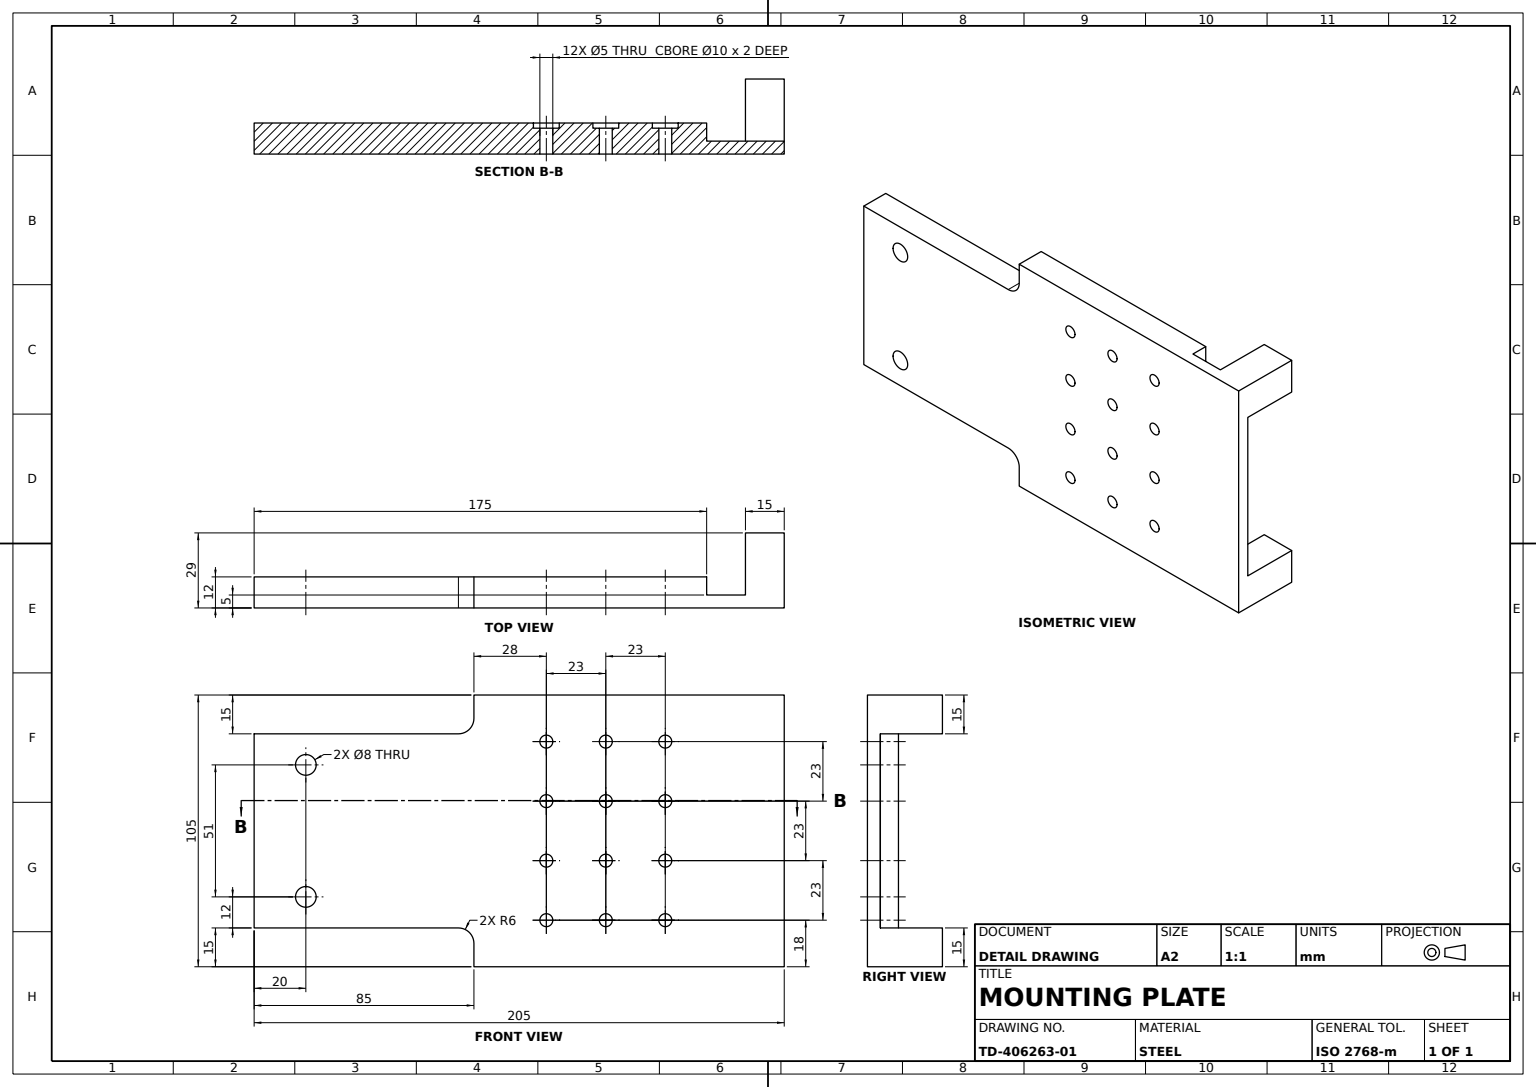
solid
v1 (154,26,2)
v2 (164,26,2)
e1 v1 v2 CIRCLE(AX(P(159,26,2),D(0,0,-1),D(-1,0,0)),5)
v3 (154,26,0)
e2 v1 v3 LINE
v4 (164,26,0)
e3 v3 v4 CIRCLE(AX(P(159,26,0),D(0,0,-1),D(-1,0,0)),5)
e4 v2 v4 LINE
face CYL(AX(P(159,26,2),D(0,0,-1),D(-1,0,0)),5) rev [-e1 e2 e3 -e4]
v5 (138.5,49,12)
v6 (138.5,49,2)
e5 v5 v6 LINE
v7 (133.5,49,12)
e6 v7 v5 CIRCLE(AX(P(136,49,12),D(0,0,-1),D(-1,0,0)),2.5)
v8 (133.5,49,2)
e7 v7 v8 LINE
e8 v8 v6 CIRCLE(AX(P(136,49,2),D(0,0,-1),D(-1,0,0)),2.5)
face CYL(AX(P(136,49,12),D(0,0,-1),D(-1,0,0)),2.5) rev [-e5 -e6 e7 e8]
v9 (138.5,72,12)
v10 (138.5,72,2)
e9 v9 v10 LINE
v11 (133.5,72,2)
e10 v10 v11 CIRCLE(AX(P(136,72,2),D(0,0,-1),D(-1,0,0)),2.5)
v12 (133.5,72,12)
e11 v12 v11 LINE
e12 v9 v12 CIRCLE(AX(P(136,72,12),D(0,0,-1),D(-1,0,0)),2.5)
face CYL(AX(P(136,72,12),D(0,0,-1),D(-1,0,0)),2.5) rev [e9 e10 -e11 -e12]
v13 (205,-15,-17)
v14 (205,-15,12)
e13 v13 v14 LINE
v15 (85,-15,12)
e14 v14 v15 LINE
v16 (85,-15,0)
e15 v16 v15 LINE
v17 (175,-15,0)
e16 v17 v16 LINE
v18 (175,-15,7)
e17 v17 v18 LINE
v19 (190,-15,7)
e18 v18 v19 LINE
v20 (190,-15,-17)
e19 v19 v20 LINE
e20 v20 v13 LINE
face PLANE(AX(P(0,-15,0),D(0,1,0),D(0,0,1))) rev [e13 e14 -e15 -e16 e17 e18 e19 e20]
v21 (16,63,12)
v22 (24,63,12)
e21 v21 v22 CIRCLE(AX(P(20,63,12),D(0,0,1),D(1,0,0)),4)
v23 (24,63,0)
e22 v22 v23 LINE
v24 (16,63,0)
e23 v23 v24 CIRCLE(AX(P(20,63,0),D(0,0,-1),D(-1,0,0)),4)
e24 v21 v24 LINE
face CYL(AX(P(20,63,15),D(0,0,-1),D(-1,0,0)),4) rev [e21 e22 e23 -e24]
v25 (108,26,0)
v26 (118,26,0)
e25 v25 v26 CIRCLE(AX(P(113,26,0),D(0,0,-1),D(-1,0,0)),5)
v27 (118,26,2)
e26 v27 v26 LINE
v28 (108,26,2)
e27 v28 v27 CIRCLE(AX(P(113,26,2),D(0,0,-1),D(-1,0,0)),5)
e28 v28 v25 LINE
face CYL(AX(P(113,26,2),D(0,0,-1),D(-1,0,0)),5) rev [e25 -e26 -e27 e28]
v29 (108,72,2)
v30 (118,72,2)
e29 v29 v30 CIRCLE(AX(P(113,72,2),D(0,0,-1),D(-1,0,0)),5)
v31 (108,72,0)
e30 v29 v31 LINE
v32 (118,72,0)
e31 v31 v32 CIRCLE(AX(P(113,72,0),D(0,0,-1),D(-1,0,0)),5)
e32 v30 v32 LINE
face CYL(AX(P(113,72,2),D(0,0,-1),D(-1,0,0)),5) rev [-e29 e30 e31 -e32]
v33 (110.5,3,12)
v34 (115.5,3,12)
e33 v33 v34 CIRCLE(AX(P(113,3,12),D(0,0,-1),D(-1,0,0)),2.5)
v35 (110.5,3,2)
e34 v33 v35 LINE
v36 (115.5,3,2)
e35 v35 v36 CIRCLE(AX(P(113,3,2),D(0,0,-1),D(-1,0,0)),2.5)
e36 v34 v36 LINE
face CYL(AX(P(113,3,12),D(0,0,-1),D(-1,0,0)),2.5) rev [-e33 e34 e35 -e36]
v37 (141,3,2)
v38 (131,3,2)
e37 v37 v38 CIRCLE(AX(P(136,3,2),D(0,0,-1),D(-1,0,0)),5)
e38 v38 v37 CIRCLE(AX(P(136,3,2),D(0,0,-1),D(-1,0,0)),5)
v39 (133.5,3,2)
v40 (138.5,3,2)
e39 v39 v40 CIRCLE(AX(P(136,3,2),D(0,0,-1),D(-1,0,0)),2.5)
e40 v40 v39 CIRCLE(AX(P(136,3,2),D(0,0,-1),D(-1,0,0)),2.5)
face PLANE(AX(P(0,0,2),D(0,0,-1),D(-1,0,0))) [e37 e38] [-e39 -e40]
e41 v5 v7 CIRCLE(AX(P(136,49,12),D(0,0,-1),D(-1,0,0)),2.5)
e42 v6 v8 CIRCLE(AX(P(136,49,2),D(0,0,-1),D(-1,0,0)),2.5)
face CYL(AX(P(136,49,12),D(0,0,-1),D(-1,0,0)),2.5) rev [-e7 -e41 e5 e42]
v41 (131,3,0)
v42 (141,3,0)
e43 v41 v42 CIRCLE(AX(P(136,3,0),D(0,0,-1),D(-1,0,0)),5)
e44 v37 v42 LINE
e45 v38 v41 LINE
face CYL(AX(P(136,3,2),D(0,0,-1),D(-1,0,0)),5) rev [e43 -e44 -e38 e45]
v43 (110.5,26,2)
v44 (115.5,26,2)
e46 v43 v44 CIRCLE(AX(P(113,26,2),D(0,0,-1),D(-1,0,0)),2.5)
e47 v44 v43 CIRCLE(AX(P(113,26,2),D(0,0,-1),D(-1,0,0)),2.5)
e48 v27 v28 CIRCLE(AX(P(113,26,2),D(0,0,-1),D(-1,0,0)),5)
face PLANE(AX(P(0,0,2),D(0,0,-1),D(-1,0,0))) [-e46 -e47] [e48 e27]
v45 (161.5,72,12)
v46 (156.5,72,12)
e49 v45 v46 CIRCLE(AX(P(159,72,12),D(0,0,-1),D(-1,0,0)),2.5)
v47 (161.5,72,2)
e50 v45 v47 LINE
v48 (156.5,72,2)
e51 v47 v48 CIRCLE(AX(P(159,72,2),D(0,0,-1),D(-1,0,0)),2.5)
e52 v46 v48 LINE
face CYL(AX(P(159,72,12),D(0,0,-1),D(-1,0,0)),2.5) rev [-e49 e50 e51 -e52]
v49 (141,26,0)
v50 (131,26,0)
e53 v49 v50 CIRCLE(AX(P(136,26,0),D(0,0,-1),D(-1,0,0)),5)
v51 (131,26,2)
e54 v51 v50 LINE
v52 (141,26,2)
e55 v52 v51 CIRCLE(AX(P(136,26,2),D(0,0,-1),D(-1,0,0)),5)
e56 v52 v49 LINE
face CYL(AX(P(136,26,2),D(0,0,-1),D(-1,0,0)),5) rev [e53 -e54 -e55 e56]
v53 (190,0,-17)
v54 (205,0,-17)
e57 v53 v54 LINE
e58 v54 v13 LINE
e59 v53 v20 LINE
face PLANE(AX(P(190,0,-17),D(0,0,-1),D(-1,0,0))) [e57 e58 -e20 -e59]
v55 (154,49,2)
v56 (164,49,2)
e60 v55 v56 CIRCLE(AX(P(159,49,2),D(0,0,-1),D(-1,0,0)),5)
e61 v56 v55 CIRCLE(AX(P(159,49,2),D(0,0,-1),D(-1,0,0)),5)
v57 (161.5,49,2)
v58 (156.5,49,2)
e62 v57 v58 CIRCLE(AX(P(159,49,2),D(0,0,-1),D(-1,0,0)),2.5)
e63 v58 v57 CIRCLE(AX(P(159,49,2),D(0,0,-1),D(-1,0,0)),2.5)
face PLANE(AX(P(0,0,2),D(0,0,-1),D(-1,0,0))) [e60 e61] [-e62 -e63]
e64 v50 v49 CIRCLE(AX(P(136,26,0),D(0,0,-1),D(-1,0,0)),5)
e65 v51 v52 CIRCLE(AX(P(136,26,2),D(0,0,-1),D(-1,0,0)),5)
face CYL(AX(P(136,26,2),D(0,0,-1),D(-1,0,0)),5) rev [e54 e64 -e56 -e65]
v59 (164,3,2)
v60 (164,3,0)
e66 v59 v60 LINE
v61 (154,3,0)
e67 v60 v61 CIRCLE(AX(P(159,3,0),D(0,0,-1),D(-1,0,0)),5)
v62 (154,3,2)
e68 v62 v61 LINE
e69 v59 v62 CIRCLE(AX(P(159,3,2),D(0,0,-1),D(-1,0,0)),5)
face CYL(AX(P(159,3,2),D(0,0,-1),D(-1,0,0)),5) rev [e66 e67 -e68 -e69]
v63 (118,3,2)
v64 (108,3,2)
e70 v63 v64 CIRCLE(AX(P(113,3,2),D(0,0,-1),D(-1,0,0)),5)
v65 (118,3,0)
e71 v63 v65 LINE
v66 (108,3,0)
e72 v65 v66 CIRCLE(AX(P(113,3,0),D(0,0,-1),D(-1,0,0)),5)
e73 v64 v66 LINE
face CYL(AX(P(113,3,2),D(0,0,-1),D(-1,0,0)),5) rev [-e70 e71 e72 -e73]
v67 (161.5,26,2)
v68 (156.5,26,2)
e74 v67 v68 CIRCLE(AX(P(159,26,2),D(0,0,-1),D(-1,0,0)),2.5)
v69 (156.5,26,12)
e75 v69 v68 LINE
v70 (161.5,26,12)
e76 v70 v69 CIRCLE(AX(P(159,26,12),D(0,0,-1),D(-1,0,0)),2.5)
e77 v70 v67 LINE
face CYL(AX(P(159,26,12),D(0,0,-1),D(-1,0,0)),2.5) rev [e74 -e75 -e76 e77]
v71 (115.5,49,12)
v72 (110.5,49,12)
e78 v71 v72 CIRCLE(AX(P(113,49,12),D(0,0,-1),D(-1,0,0)),2.5)
v73 (115.5,49,2)
e79 v71 v73 LINE
v74 (110.5,49,2)
e80 v73 v74 CIRCLE(AX(P(113,49,2),D(0,0,-1),D(-1,0,0)),2.5)
e81 v72 v74 LINE
face CYL(AX(P(113,49,12),D(0,0,-1),D(-1,0,0)),2.5) rev [-e78 e79 e80 -e81]
e82 v11 v10 CIRCLE(AX(P(136,72,2),D(0,0,-1),D(-1,0,0)),2.5)
e83 v12 v9 CIRCLE(AX(P(136,72,12),D(0,0,-1),D(-1,0,0)),2.5)
face CYL(AX(P(136,72,12),D(0,0,-1),D(-1,0,0)),2.5) rev [e82 -e9 -e83 e11]
v75 (205,75,-17)
v76 (190,75,-17)
e84 v75 v76 LINE
v77 (205,75,7)
e85 v77 v75 LINE
v78 (190,75,7)
e86 v78 v77 LINE
e87 v76 v78 LINE
face PLANE(AX(P(0,75,0),D(0,-1,0),D(0,0,-1))) [-e84 -e85 -e86 -e87]
v79 (79,75,12)
v80 (0,75,12)
e88 v79 v80 LINE
v81 (79,75,0)
e89 v79 v81 LINE
v82 (0,75,0)
e90 v81 v82 LINE
e91 v80 v82 LINE
face PLANE(AX(P(85,75,12),D(0,-1,0),D(0,0,-1))) rev [-e88 e89 e90 -e91]
v83 (164,49,0)
v84 (154,49,0)
e92 v83 v84 CIRCLE(AX(P(159,49,0),D(0,0,-1),D(-1,0,0)),5)
e93 v55 v84 LINE
e94 v56 v83 LINE
face CYL(AX(P(159,49,2),D(0,0,-1),D(-1,0,0)),5) rev [e92 -e93 -e61 e94]
v85 (85,-6,0)
e95 v85 v16 LINE
v86 (85,-6,12)
e96 v86 v15 LINE
e97 v86 v85 LINE
face PLANE(AX(P(85,0,0),D(-1,0,0),D(0,0,1))) [e95 e15 -e96 e97]
v87 (110.5,72,12)
v88 (115.5,72,12)
e98 v87 v88 CIRCLE(AX(P(113,72,12),D(0,0,-1),D(-1,0,0)),2.5)
v89 (110.5,72,2)
e99 v87 v89 LINE
v90 (115.5,72,2)
e100 v89 v90 CIRCLE(AX(P(113,72,2),D(0,0,-1),D(-1,0,0)),2.5)
e101 v88 v90 LINE
face CYL(AX(P(113,72,12),D(0,0,-1),D(-1,0,0)),2.5) rev [-e98 e99 e100 -e101]
e102 v74 v73 CIRCLE(AX(P(113,49,2),D(0,0,-1),D(-1,0,0)),2.5)
e103 v72 v71 CIRCLE(AX(P(113,49,12),D(0,0,-1),D(-1,0,0)),2.5)
face CYL(AX(P(113,49,12),D(0,0,-1),D(-1,0,0)),2.5) rev [e102 -e79 -e103 e81]
v91 (156.5,3,12)
v92 (156.5,3,2)
e104 v91 v92 LINE
v93 (161.5,3,12)
e105 v93 v91 CIRCLE(AX(P(159,3,12),D(0,0,-1),D(-1,0,0)),2.5)
v94 (161.5,3,2)
e106 v93 v94 LINE
e107 v94 v92 CIRCLE(AX(P(159,3,2),D(0,0,-1),D(-1,0,0)),2.5)
face CYL(AX(P(159,3,12),D(0,0,-1),D(-1,0,0)),2.5) rev [-e104 -e105 e106 e107]
e108 v30 v29 CIRCLE(AX(P(113,72,2),D(0,0,-1),D(-1,0,0)),5)
e109 v90 v89 CIRCLE(AX(P(113,72,2),D(0,0,-1),D(-1,0,0)),2.5)
face PLANE(AX(P(0,0,2),D(0,0,-1),D(-1,0,0))) [e29 e108] [-e109 -e100]
v95 (85,90,0)
v96 (85,81,0)
e110 v95 v96 LINE
v97 (85,81,12)
e111 v96 v97 LINE
v98 (85,90,12)
e112 v98 v97 LINE
e113 v95 v98 LINE
face PLANE(AX(P(85,0,0),D(-1,0,0),D(0,0,1))) [e110 e111 -e112 -e113]
e114 v64 v63 CIRCLE(AX(P(113,3,2),D(0,0,-1),D(-1,0,0)),5)
e115 v66 v65 CIRCLE(AX(P(113,3,0),D(0,0,-1),D(-1,0,0)),5)
face CYL(AX(P(113,3,2),D(0,0,-1),D(-1,0,0)),5) rev [-e71 -e114 e73 e115]
v99 (190,90,7)
e116 v78 v99 LINE
v100 (190,90,-17)
e117 v100 v99 LINE
e118 v76 v100 LINE
face PLANE(AX(P(190,75,7),D(-1,0,0),D(0,0,1))) [e87 e116 -e117 -e118]
e119 v22 v21 CIRCLE(AX(P(20,63,12),D(0,0,1),D(1,0,0)),4)
e120 v24 v23 CIRCLE(AX(P(20,63,0),D(0,0,-1),D(-1,0,0)),4)
face CYL(AX(P(20,63,15),D(0,0,-1),D(-1,0,0)),4) rev [e119 e24 e120 -e22]
e121 v92 v94 CIRCLE(AX(P(159,3,2),D(0,0,-1),D(-1,0,0)),2.5)
e122 v62 v59 CIRCLE(AX(P(159,3,2),D(0,0,-1),D(-1,0,0)),5)
face PLANE(AX(P(0,0,2),D(0,0,-1),D(-1,0,0))) [-e107 -e121] [e122 e69]
v101 (118,49,0)
v102 (108,49,0)
e123 v101 v102 CIRCLE(AX(P(113,49,0),D(0,0,-1),D(-1,0,0)),5)
v103 (108,49,2)
e124 v103 v102 LINE
v104 (118,49,2)
e125 v104 v103 CIRCLE(AX(P(113,49,2),D(0,0,-1),D(-1,0,0)),5)
e126 v104 v101 LINE
face CYL(AX(P(113,49,2),D(0,0,-1),D(-1,0,0)),5) rev [e123 -e124 -e125 e126]
e127 v2 v1 CIRCLE(AX(P(159,26,2),D(0,0,-1),D(-1,0,0)),5)
e128 v68 v67 CIRCLE(AX(P(159,26,2),D(0,0,-1),D(-1,0,0)),2.5)
face PLANE(AX(P(0,0,2),D(0,0,-1),D(-1,0,0))) [e1 e127] [-e128 -e74]
v105 (156.5,49,12)
e129 v105 v58 LINE
v106 (161.5,49,12)
e130 v106 v105 CIRCLE(AX(P(159,49,12),D(0,0,-1),D(-1,0,0)),2.5)
e131 v106 v57 LINE
face CYL(AX(P(159,49,12),D(0,0,-1),D(-1,0,0)),2.5) rev [-e129 -e130 e131 e62]
v107 (133.5,26,12)
v108 (133.5,26,2)
e132 v107 v108 LINE
v109 (138.5,26,12)
e133 v109 v107 CIRCLE(AX(P(136,26,12),D(0,0,-1),D(-1,0,0)),2.5)
v110 (138.5,26,2)
e134 v109 v110 LINE
e135 v110 v108 CIRCLE(AX(P(136,26,2),D(0,0,-1),D(-1,0,0)),2.5)
face CYL(AX(P(136,26,12),D(0,0,-1),D(-1,0,0)),2.5) rev [-e132 -e133 e134 e135]
v111 (164,72,0)
v112 (154,72,0)
e136 v111 v112 CIRCLE(AX(P(159,72,0),D(0,0,-1),D(-1,0,0)),5)
e137 v112 v111 CIRCLE(AX(P(159,72,0),D(0,0,-1),D(-1,0,0)),5)
e138 v102 v101 CIRCLE(AX(P(113,49,0),D(0,0,-1),D(-1,0,0)),5)
v113 (0,0,0)
e139 v82 v113 LINE
e140 v81 v96 CIRCLE(AX(P(79,81,0),D(0,0,1),D(1,0,0)),6)
v114 (175,90,0)
e141 v114 v95 LINE
e142 v17 v114 LINE
v115 (79,0,0)
e143 v85 v115 CIRCLE(AX(P(79,-6,0),D(0,0,1),D(1,0,0)),6)
e144 v113 v115 LINE
e145 v4 v3 CIRCLE(AX(P(159,26,0),D(0,0,-1),D(-1,0,0)),5)
v116 (141,49,0)
v117 (131,49,0)
e146 v116 v117 CIRCLE(AX(P(136,49,0),D(0,0,-1),D(-1,0,0)),5)
e147 v117 v116 CIRCLE(AX(P(136,49,0),D(0,0,-1),D(-1,0,0)),5)
v118 (24,12,0)
v119 (16,12,0)
e148 v118 v119 CIRCLE(AX(P(20,12,0),D(0,0,-1),D(-1,0,0)),4)
e149 v119 v118 CIRCLE(AX(P(20,12,0),D(0,0,-1),D(-1,0,0)),4)
e150 v61 v60 CIRCLE(AX(P(159,3,0),D(0,0,-1),D(-1,0,0)),5)
e151 v84 v83 CIRCLE(AX(P(159,49,0),D(0,0,-1),D(-1,0,0)),5)
e152 v42 v41 CIRCLE(AX(P(136,3,0),D(0,0,-1),D(-1,0,0)),5)
e153 v32 v31 CIRCLE(AX(P(113,72,0),D(0,0,-1),D(-1,0,0)),5)
v120 (141,72,0)
v121 (131,72,0)
e154 v120 v121 CIRCLE(AX(P(136,72,0),D(0,0,-1),D(-1,0,0)),5)
e155 v121 v120 CIRCLE(AX(P(136,72,0),D(0,0,-1),D(-1,0,0)),5)
e156 v26 v25 CIRCLE(AX(P(113,26,0),D(0,0,-1),D(-1,0,0)),5)
face PLANE(AX(P(0,0,0),D(0,0,1),D(1,0,0))) rev [-e53 -e64] [-e136 -e137] [-e138 -e123] [-e72 -e115] [-e139 -e90 e140 -e110 -e141 -e142 e16 -e95 e143 -e144] [-e3 -e145] [-e146 -e147] [-e148 -e149] [-e67 -e150] [-e151 -e92] [-e23 -e120] [-e43 -e152] [-e153 -e31] [-e154 -e155] [-e25 -e156]
v122 (133.5,3,12)
e157 v122 v39 LINE
v123 (138.5,3,12)
e158 v123 v122 CIRCLE(AX(P(136,3,12),D(0,0,-1),D(-1,0,0)),2.5)
e159 v123 v40 LINE
face CYL(AX(P(136,3,12),D(0,0,-1),D(-1,0,0)),2.5) rev [e40 -e157 -e158 e159]
e160 v91 v93 CIRCLE(AX(P(159,3,12),D(0,0,-1),D(-1,0,0)),2.5)
face CYL(AX(P(159,3,12),D(0,0,-1),D(-1,0,0)),2.5) rev [e121 -e106 -e160 e104]
v124 (79,0,12)
e161 v115 v124 LINE
v125 (0,0,12)
e162 v125 v124 LINE
e163 v125 v113 LINE
face PLANE(AX(P(0,0,12),D(0,1,0),D(0,0,1))) rev [e161 -e162 e163 e144]
v126 (164,72,2)
e164 v126 v111 LINE
v127 (154,72,2)
e165 v127 v112 LINE
e166 v126 v127 CIRCLE(AX(P(159,72,2),D(0,0,-1),D(-1,0,0)),5)
face CYL(AX(P(159,72,2),D(0,0,-1),D(-1,0,0)),5) rev [e164 e136 -e165 -e166]
e167 v105 v106 CIRCLE(AX(P(159,49,12),D(0,0,-1),D(-1,0,0)),2.5)
face CYL(AX(P(159,49,12),D(0,0,-1),D(-1,0,0)),2.5) rev [-e131 -e167 e129 e63]
face CYL(AX(P(159,3,2),D(0,0,-1),D(-1,0,0)),5) rev [-e122 e68 e150 -e66]
v128 (205,90,-17)
e168 v128 v100 LINE
v129 (175,90,7)
e169 v99 v129 LINE
e170 v114 v129 LINE
v130 (205,90,12)
e171 v130 v98 LINE
e172 v128 v130 LINE
face PLANE(AX(P(0,90,0),D(0,1,0),D(0,0,1))) [e168 e117 e169 -e170 e141 e113 -e171 -e172]
e173 v88 v87 CIRCLE(AX(P(113,72,12),D(0,0,-1),D(-1,0,0)),2.5)
face CYL(AX(P(113,72,12),D(0,0,-1),D(-1,0,0)),2.5) rev [e101 e109 -e99 -e173]
v131 (190,0,7)
e174 v131 v19 LINE
e175 v131 v53 LINE
face PLANE(AX(P(190,0,7),D(-1,0,0),D(0,0,1))) [e59 -e19 -e174 e175]
v132 (24,12,12)
v133 (16,12,12)
e176 v132 v133 CIRCLE(AX(P(20,12,12),D(0,0,1),D(1,0,0)),4)
e177 v133 v119 LINE
e178 v132 v118 LINE
face CYL(AX(P(20,12,15),D(0,0,-1),D(-1,0,0)),4) rev [e176 e177 e149 -e178]
e179 v108 v110 CIRCLE(AX(P(136,26,2),D(0,0,-1),D(-1,0,0)),2.5)
face PLANE(AX(P(0,0,2),D(0,0,-1),D(-1,0,0))) [e65 e55] [-e135 -e179]
v134 (141,49,2)
e180 v134 v116 LINE
v135 (131,49,2)
e181 v135 v134 CIRCLE(AX(P(136,49,2),D(0,0,-1),D(-1,0,0)),5)
e182 v135 v117 LINE
face CYL(AX(P(136,49,2),D(0,0,-1),D(-1,0,0)),5) rev [e147 -e180 -e181 e182]
e183 v103 v104 CIRCLE(AX(P(113,49,2),D(0,0,-1),D(-1,0,0)),5)
face PLANE(AX(P(0,0,2),D(0,0,-1),D(-1,0,0))) [-e80 -e102] [e125 e183]
e184 v127 v126 CIRCLE(AX(P(159,72,2),D(0,0,-1),D(-1,0,0)),5)
e185 v48 v47 CIRCLE(AX(P(159,72,2),D(0,0,-1),D(-1,0,0)),2.5)
face PLANE(AX(P(0,0,2),D(0,0,-1),D(-1,0,0))) [e184 e166] [-e51 -e185]
face CYL(AX(P(113,72,2),D(0,0,-1),D(-1,0,0)),5) rev [-e108 e32 e153 -e30]
v136 (141,72,2)
v137 (131,72,2)
e186 v136 v137 CIRCLE(AX(P(136,72,2),D(0,0,-1),D(-1,0,0)),5)
e187 v137 v136 CIRCLE(AX(P(136,72,2),D(0,0,-1),D(-1,0,0)),5)
face PLANE(AX(P(0,0,2),D(0,0,-1),D(-1,0,0))) [-e10 -e82] [e186 e187]
e188 v46 v45 CIRCLE(AX(P(159,72,12),D(0,0,-1),D(-1,0,0)),2.5)
face CYL(AX(P(159,72,12),D(0,0,-1),D(-1,0,0)),2.5) rev [-e188 e52 e185 -e50]
e189 v122 v123 CIRCLE(AX(P(136,3,12),D(0,0,-1),D(-1,0,0)),2.5)
face CYL(AX(P(136,3,12),D(0,0,-1),D(-1,0,0)),2.5) rev [e157 e39 -e159 -e189]
e190 v97 v79 CIRCLE(AX(P(79,81,12),D(0,0,-1),D(1,0,0)),6)
face CYL(AX(P(79,81,12),D(0,0,-1),D(-1,0,0)),6) rev [-e190 -e111 -e140 -e89]
e191 v137 v121 LINE
e192 v136 v120 LINE
face CYL(AX(P(136,72,2),D(0,0,-1),D(-1,0,0)),5) rev [e154 -e191 -e186 e192]
face CYL(AX(P(159,26,2),D(0,0,-1),D(-1,0,0)),5) rev [e4 e145 -e2 -e127]
e193 v14 v130 LINE
v138 (205,0,7)
e194 v54 v138 LINE
e195 v138 v77 LINE
e196 v75 v128 LINE
face PLANE(AX(P(205,90,7),D(1,0,0),D(0,0,-1))) [-e193 -e13 -e58 e194 e195 e85 e196 e172]
e197 v129 v18 LINE
face PLANE(AX(P(175,0,0),D(1,0,0),D(0,0,-1))) [e142 e170 e197 -e17]
v139 (110.5,26,12)
e198 v139 v43 LINE
v140 (115.5,26,12)
e199 v140 v139 CIRCLE(AX(P(113,26,12),D(0,0,-1),D(-1,0,0)),2.5)
e200 v140 v44 LINE
face CYL(AX(P(113,26,12),D(0,0,-1),D(-1,0,0)),2.5) rev [-e198 -e199 e200 e47]
face CYL(AX(P(113,26,2),D(0,0,-1),D(-1,0,0)),5) rev [-e28 -e48 e26 e156]
face CYL(AX(P(159,72,2),D(0,0,-1),D(-1,0,0)),5) rev [-e164 -e184 e165 e137]
e201 v36 v35 CIRCLE(AX(P(113,3,2),D(0,0,-1),D(-1,0,0)),2.5)
e202 v34 v33 CIRCLE(AX(P(113,3,12),D(0,0,-1),D(-1,0,0)),2.5)
face CYL(AX(P(113,3,12),D(0,0,-1),D(-1,0,0)),2.5) rev [e36 e201 -e34 -e202]
e203 v124 v86 CIRCLE(AX(P(79,-6,12),D(0,0,-1),D(1,0,0)),6)
face CYL(AX(P(79,-6,0),D(0,0,-1),D(-1,0,0)),6) rev [-e97 -e203 -e161 -e143]
face PLANE(AX(P(0,0,2),D(0,0,-1),D(-1,0,0))) [-e35 -e201] [e114 e70]
e204 v134 v135 CIRCLE(AX(P(136,49,2),D(0,0,-1),D(-1,0,0)),5)
face PLANE(AX(P(0,0,2),D(0,0,-1),D(-1,0,0))) [-e8 -e42] [e204 e181]
face CYL(AX(P(159,49,2),D(0,0,-1),D(-1,0,0)),5) rev [e93 e151 -e94 -e60]
e205 v69 v70 CIRCLE(AX(P(159,26,12),D(0,0,-1),D(-1,0,0)),2.5)
e206 v133 v132 CIRCLE(AX(P(20,12,12),D(0,0,1),D(1,0,0)),4)
e207 v107 v109 CIRCLE(AX(P(136,26,12),D(0,0,-1),D(-1,0,0)),2.5)
e208 v80 v125 LINE
e209 v139 v140 CIRCLE(AX(P(113,26,12),D(0,0,-1),D(-1,0,0)),2.5)
face PLANE(AX(P(0,0,12),D(0,0,1),D(1,0,0))) [e76 e205] [e188 e49] [e12 e83] [e105 e160] [e41 e6] [e173 e98] [e78 e103] [-e21 -e119] [-e176 -e206] [e130 e167] [e202 e33] [e207 e133] [e162 e203 e96 -e14 e193 e171 e112 e190 e88 e208] [e189 e158] [e209 e199]
face CYL(AX(P(159,26,12),D(0,0,-1),D(-1,0,0)),2.5) rev [-e205 e75 e128 -e77]
face CYL(AX(P(136,26,12),D(0,0,-1),D(-1,0,0)),2.5) rev [-e207 e132 e179 -e134]
face CYL(AX(P(136,49,2),D(0,0,-1),D(-1,0,0)),5) rev [e146 -e182 -e204 e180]
face CYL(AX(P(136,72,2),D(0,0,-1),D(-1,0,0)),5) rev [e155 -e192 -e187 e191]
face CYL(AX(P(113,26,12),D(0,0,-1),D(-1,0,0)),2.5) rev [-e209 e198 e46 -e200]
face PLANE(AX(P(0,75,12),D(1,0,0),D(0,0,-1))) rev [-e208 e91 e139 -e163]
face CYL(AX(P(136,3,2),D(0,0,-1),D(-1,0,0)),5) rev [e44 e152 -e45 -e37]
face CYL(AX(P(20,12,15),D(0,0,-1),D(-1,0,0)),4) rev [-e177 e206 e178 e148]
e210 v138 v131 LINE
face PLANE(AX(P(0,0,0),D(0,-1,0),D(0,0,-1))) rev [-e194 -e57 -e175 -e210]
face PLANE(AX(P(0,0,7),D(0,0,-1),D(-1,0,0))) [e210 e174 -e18 -e197 -e169 -e116 e86 -e195]
face CYL(AX(P(113,49,2),D(0,0,-1),D(-1,0,0)),5) rev [e138 -e126 -e183 e124]
face PLANE(AX(P(190,75,-17),D(0,0,-1),D(-1,0,0))) [e84 e118 -e168 -e196]
